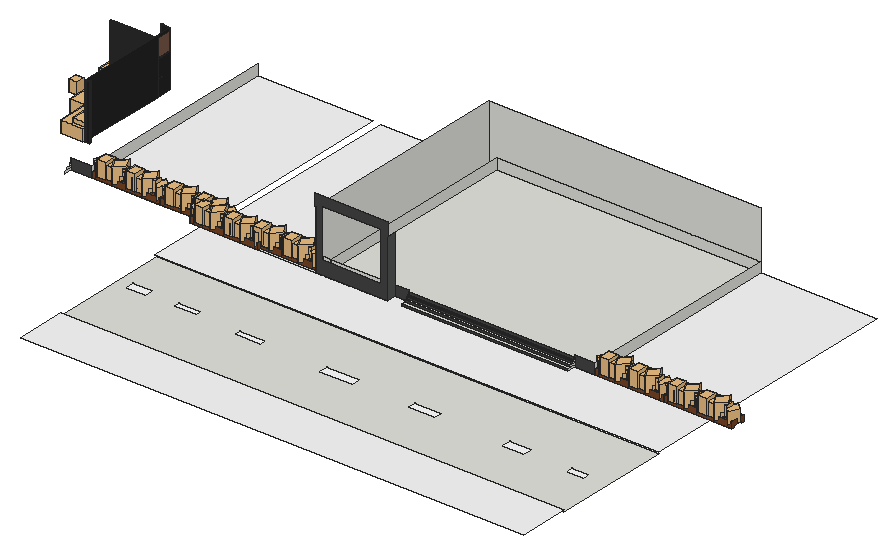
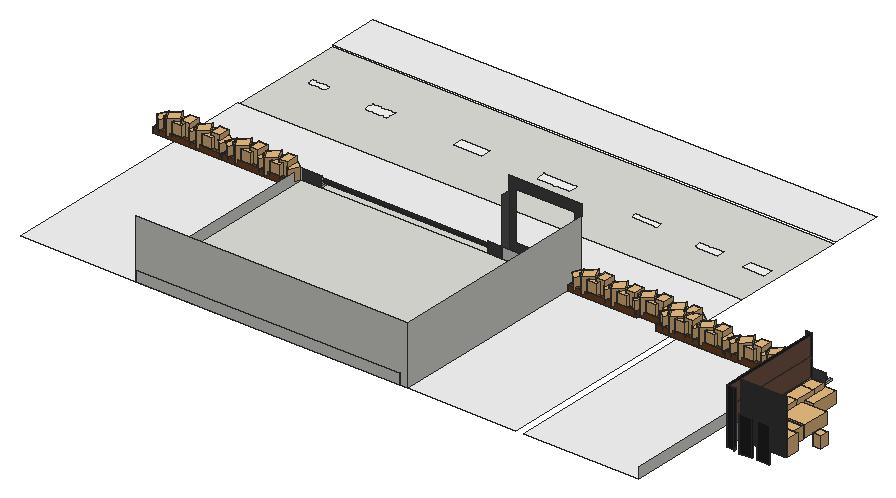
# SketchUp Ruby script. Lengths in inches.
U = 1.inch
M = Sketchup.active_model
def pt(a) = Geom::Point3d.new(a.map { |v| v * U })
def face(e, loops, mat)
  f = e.add_face(loops[0].map { |a| pt(a) })
  loops[1..].each { |l| e.add_face(l.map { |a| pt(a) }).erase! }
  f.material = f.back_material = mat if mat
  f
end
# faces: each face lists its corners as indices into pts; further lists are holes
def faces(e, pts, list, mat = nil) = list.each { |f| face(e, (f[0].is_a?(Array) ? f : [f]).map { |l| l.map { |i| pts[i] } }, mat) }
# xy, xz, yz: faces in a plane at the given z, y or x. An outline is a flat list of corners, or four numbers for a rectangle; further outlines are holes
def ring(l) = l.size == 4 ? [[l[0], l[1]], [l[2], l[1]], [l[2], l[3]], [l[0], l[3]]] : l.each_slice(2).to_a
def flat(e, list, mat, &to3) = list.each { |f| face(e, (f[0].is_a?(Array) ? f : [f]).map { |l| ring(l).map { |u, v| to3.(u, v) } }, mat) }
def xy(e, z, list, mat = nil) = flat(e, list, mat) { |x, y| [x, y, z] }
def xz(e, y, list, mat = nil) = flat(e, list, mat) { |x, z| [x, y, z] }
def yz(e, x, list, mat = nil) = flat(e, list, mat) { |y, z| [x, y, z] }
def lines(e, pts, list) = list.each { |a, b| e.add_line(pt(pts[a]), pt(pts[b])) }
# prism: a flat outline (further loops are holes) pulled along v
def prism(e, loops, v, mat = nil)
  f = face(e, loops, mat); d = Geom::Vector3d.new(v.map { |x| x * U })
  f.pushpull(f.normal.samedirection?(d) ? d.length : -d.length)
end
def box(e, o, s, mat = nil) = prism(e, [[o, [o[0] + s[0], o[1], o[2]], [o[0] + s[0], o[1] + s[1], o[2]], [o[0], o[1] + s[1], o[2]]]], [0, 0, s[2]], mat)
def at(x, y, z, deg = 0) = Geom::Transformation.translation(pt([x, y, z])) * Geom::Transformation.rotation(ORIGIN, Z_AXIS, deg.degrees)
def axes(o, x, y, z) = Geom::Transformation.new([*x, 0, *y, 0, *z, 0, *pt(o).to_a, 1])
def part(name) = M.definitions.add(name)
# library, detail: a bought-in or finely detailed component or shape, given as its bounding box
def library(name, o, s) = part(name).tap { |d| box(d.entities, o, s) }
def detail(e, o, s) = box(e.add_group.entities, o, s)
def put(e, d, t, mat = nil) = e.add_instance(d, t).tap { |i| i.material = mat if mat }
def group(e, t, mat = nil) = e.add_group.tap { |g| g.transformation = t; g.material = mat if mat }.entities
root = M.entities
M.materials.add("Aluminum_Polished").color = [83, 85, 85]
M.materials.add("Color_").color = [255, 255, 255]
M.materials.add("Floor board").color = [119, 86, 70]
M.materials.add("Floor board2").color = [119, 86, 70]
M.materials.add("Material__1").color = [95, 70, 46]
M.materials.add("Screen Shot 2014-10-30 at 12.13.07").color = [162, 155, 149]
M.materials.add("Sophie_Shoes2").color = [35, 35, 35]
M.materials.add("Untitsled-1").color = [96, 91, 93]
M.materials.add("Wood_Grain_Dark").color = [51, 47, 43]
M.materials.add("[Granite Dark Gray]").color = [69, 68, 68]
M.materials.add("[Metal_Corrogated_Shiny]2").color = [193, 193, 193]
M.materials.add("[Tile Grey]").color = [249, 249, 249]
M.materials.add("[Wood Veneer 01]").color = [120, 70, 37]
c1 = library("ch24 wishbone chair by Carl Hansen & Son",[0,0,0],[21.1,19.68,29.02])
c2 = part("Group\#72")
box(c2.entities,[0,-0.59,0],[31.5,1.77,87.4],"Sophie_Shoes2")
c3 = library("Armless sofa",[0,0,0],[31.59,51.18,39.76])
c4 = library("Sofa corner unit",[0,0,0],[31.57,31.52,39.76])
c5 = part("Group\#13")
box(c5.entities,[-0.79,0,0],[1.97,3.15,131.5],"Wood_Grain_Dark")
c6 = library("Group\#91",[-37.8,-0.03,0],[93.74,69.5,29.53])
c7 = library("Group\#68",[-37.8,-0.03,0],[93.74,69.5,29.53])
c8 = library("Group\#95",[0,-0.03,0],[55.94,69.5,29.53])
c9 = library("Areca palm plant",[0,0,0],[49.1,36.6,54.46])
c10 = library("Group\#440",[-84.69,-90.07,-0.36],[176.51,175.13,171.4])
c11 = library("Group\#441",[-7.34,-1.2,0],[38.67,35.81,49.04])
c12 = library("Group38\#2",[14.01,28.44,-23.43],[18.58,18.32,38.89])
c13 = library("Group20\#1",[-20.81,-17.08,3.79],[39.86,39.43,37.51])
c14 = part("Group\#443")
put(c14.entities,c9,axes([76.39,-6.2,6.08],[0.56191,0.45017,0],[-0.52986,0.66137,0],[0,0,0.72]))
put(c14.entities,c9,axes([178.2,-6.2,6.08],[0.56191,0.45017,0],[-0.52986,0.66137,0],[0,0,0.72]))
put(c14.entities,c10,axes([163.5,14.93,6.05],[0.08593,-0.04961,0],[0.04961,0.08593,0],[0,0,0.10522]))
put(c14.entities,c11,axes([144.89,24.9375,8],[-0.79,0,0],[0,-0.79,0],[0,0,0.79]))
put(c14.entities,c10,axes([113.57,17.19,6.07],[0.14087,-0.08133,0],[0.08133,0.14087,0],[0,0,0.1725]))
put(c14.entities,c12,axes([235.95,-4.1,28.17],[0,0.8848,0],[-0.94674,0,0],[0,0,0.85826]))
put(c14.entities,c10,axes([190.75,14.93,6.05],[0.08593,-0.04961,0],[0.04961,0.08593,0],[0,0,0.10522]))
put(c14.entities,c10,axes([61.68,14.93,6.05],[0.08593,-0.04961,0],[0.04961,0.08593,0],[0,0,0.10522]))
put(c14.entities,c10,axes([88.93,14.93,6.05],[0.08593,-0.04961,0],[0.04961,0.08593,0],[0,0,0.10522]))
put(c14.entities,c13,axes([154.82,18.97,4.77],[-0.85,0,0],[0,-0.85,0],[0,0,0.85]))
put(c14.entities,c10,axes([41.62,14.93,6.05],[0.08593,-0.04961,0],[0.04961,0.08593,0],[0,0,0.10522]))
put(c14.entities,c10,axes([143.43,14.93,6.05],[0.08593,-0.04961,0],[0.04961,0.08593,0],[0,0,0.10522]))
put(c14.entities,c12,axes([134.14,-4.1,28.17],[0,0.8848,0],[-0.94674,0,0],[0,0,0.85826]))
g1 = group(c14.entities,at(234.8,0,0,90),"[Wood Veneer 01]")
xy(g1,0,[[0,0,6,234.8],[30,0,36,234.8]])
xy(g1,3,[[6,0,30,234.8]])
xy(g1,7,[[6,5,30,229.8]],"Material__1")
xy(g1,15,[[[0,0,36,234.8],[6,5,30,229.8]]])
xz(g1,0,[[0,0,6,0,6,3,30,3,30,0,36,0,36,15,0,15]])
xz(g1,5,[[6,7,30,15]])
xz(g1,229.8,[[6,7,30,15]])
xz(g1,234.8,[[0,0,0,15,36,15,36,0,30,0,30,3,6,3,6,0]])
yz(g1,0,[[0,0,234.8,15]])
yz(g1,6,[[0,0,234.8,3],[5,7,229.8,15]])
yz(g1,30,[[0,0,234.8,3],[5,7,229.8,15]])
yz(g1,36,[[0,0,234.8,15]])
put(c14.entities,c11,axes([43.08,24.9375,8],[-0.79,0,0],[0,-0.79,0],[0,0,0.79]))
put(c14.entities,c10,axes([11.76,17.19,6.07],[0.14087,-0.08133,0],[0.08133,0.14087,0],[0,0,0.1725]))
put(c14.entities,c13,axes([53.01,18.97,4.77],[-0.85,0,0],[0,-0.85,0],[0,0,0.85]))
put(c14.entities,c10,axes([219.01,17.19,6.07],[0.14087,-0.08133,0],[0.08133,0.14087,0],[0,0,0.1725]))
c15 = part("Untitled (5)")
xy(c15.entities,0,[[[158.81,26.5625,306.06,993.3125],[226.57,518.17,239.57,583.92],[225.28,357.51,237.28,411.51],[222.61,182.28,236.36,226.53],[239.71,931.55,251.46,972.3],[233.64,703.93,242.14,755.18],[240.05,835.03,248.8,880.53],[222.04,66.5,231.29,100.5]]])
xy(c15.entities,0,[[222.04,66.5,231.29,100.5],[222.61,182.28,236.36,226.53],[225.28,357.51,237.28,411.51],[226.57,518.17,239.57,583.92],[233.64,703.93,242.14,755.18],
  [240.05,835.03,248.8,880.53],[239.71,931.55,251.46,972.3]],"Color_")
xy(root,-20.5,[[3778.5,559.875,4065.56,581.125],[4065.56,559.875,4244.09,581.125],[4279.08,559.875,4690.96,581.125],[4065.56,581.125,4085.31,1096.5],[4085.31,581.125,4742.06,1096.5]])
xy(root,-20.5,[[3778.5,419.4375,5029.12,419.4375,5029.12,581.125,4690.96,581.125,4690.96,559.875,4279.08,559.875,4279.08,581.125,4244.09,581.125,4244.09,559.875,3778.5,559.875],[3491.44,581.125,3778.5,1096.5],[3798.25,581.125,4065.56,1096.5],[4742.06,581.125,5029.12,1096.5]],"[Tile Grey]")
xy(root,-20.25,[[3778.5,0,5029.12,126.25]],"[Tile Grey]")
xy(root,-15.38,[[4279.08,559.875,4690.96,568.25]])
xy(root,-10.73,[[4279.08,568.25,4690.96,575.4375]])
xy(root,-6.62,[[4279.08,575.4375,4690.96,578]])
xy(root,-3.61,[[4279.08,578,4690.96,580.3125]])
xz(root,559.875,[[[4065.56,-20.5,4244.09,-20.5,4244.09,155.3125,4061.87,155.3125,4061.87,126,4065.56,126],[4079.48,11.5,4226.29,132]],[4279.08,-20.5,4690.96,-15.38]],"[Granite Dark Gray]")
xz(root,568.25,[[4279.08,-15.38,4690.96,-10.73]],"[Granite Dark Gray]")
xz(root,575.4375,[[4279.08,-10.73,4690.96,-6.62]],"[Granite Dark Gray]")
xz(root,578,[[4279.08,-6.62,4690.96,-3.61]],"[Granite Dark Gray]")
xz(root,580.3125,[[4279.08,-3.61,4690.96,1.19]],"[Granite Dark Gray]")
xz(root,581.125,[[4065.56,-20.5,4085.31,6],[4085.31,-20.5,4244.09,6]])
xz(root,581.125,[[3440.34,-20.5,3491.44,6],[4244.09,-20.5,4279.08,6],[4690.96,-20.5,4742.06,6]],"[Granite Dark Gray]")
xz(root,1096.5,[[4065.56,-20.5,4065.56,126,4742.06,126,4742.06,6,4085.31,6,4085.31,-20.5],[4085.31,-20.5,4742.06,6]])
yz(root,3440.34,[[559.875,-20.5,581.125,-15.38],[568.25,-15.38,581.125,-10.73],[575.4375,-10.73,581.125,-6.62],[578,-6.62,581.125,-3.61],[580.3125,-3.61,581.125,1.19]])
yz(root,3491.44,[[581.125,-20.5,1096.5,6]])
yz(root,4065.56,[[559.875,-20.5,581.125,6],[581.125,-20.5,581.125,6,559.875,6,559.875,126,1096.5,126,1096.5,-20.5]])
yz(root,4085.31,[[581.125,-20.5,1096.5,6]])
yz(root,4244.09,[[559.875,-20.5,581.125,120.25]],"Aluminum_Polished")
yz(root,4279.08,[[559.875,-20.5,581.125,-15.38],[568.25,-15.38,581.125,-10.73],[575.4375,-10.73,581.125,-6.62],[578,-6.62,581.125,-3.61],[580.3125,-3.61,581.125,1.19]])
yz(root,4690.96,[[559.875,-20.5,581.125,-15.38],[568.25,-15.38,581.125,-10.73],[575.4375,-10.73,581.125,-6.62],[578,-6.62,581.125,-3.61],[580.3125,-3.61,581.125,1.19]])
yz(root,4742.06,[[581.125,-20.5,1096.5,6]])
p = [[3345.91,994.6,0],[3345.91,994.79,0],[3427.37,658.2,0],[3427.4,658.2,0],[3414.37,657.34,0],[3414.37,657.34,86.61]]
lines(root,p,[[0,1],[2,3],[4,5]])
put(root,c1,axes([3266.16,790.81,0],[-0.00287,1,0],[1,0.00287,0],[0,0,1]))
put(root,c2,at(3304.21,923.74,0))
g2 = group(root,at(3325.58,648.625,-0.2))
put(g2,c3,at(86.72,196.88,0,-180))
put(g2,c3,at(86.72,145.7,0,-180))
put(g2,c3,at(4.02,228.45,0,-90))
put(g2,c4,at(55.2,228.45,0,-90))
put(g2,c4,at(86.72,43.34,0,-180))
put(g2,c4,at(-27.56,196.93,0))
put(g2,c3,at(86.72,94.52,0,-180))
g3 = group(root,at(3302.98,877.28,0))
put(g3,c5,at(100,0,0))
put(g3,c5,at(57.48,0,0))
put(g3,c5,at(92.91,0,0))
put(g3,c5,at(7.875,0,0))
put(g3,c5,at(107.09,0,0))
put(g3,c5,at(103.54,0,0))
put(g3,c5,at(61.02,0,0))
put(g3,c5,at(29.13,0,0))
put(g3,c5,at(68.11,0,0))
put(g3,c5,at(22.05,0,0))
put(g3,c5,at(78.74,0,0))
put(g3,c5,at(14.96,0,0))
put(g3,c5,at(82.28,0,0))
put(g3,c5,at(71.65,0,0))
put(g3,c5,at(75.2,0,0))
put(g3,c5,at(25.59,0,0))
put(g3,c5,at(18.5,0,0))
put(g3,c5,at(43.31,0,0))
put(g3,c5,at(64.57,0,0))
put(g3,c5,at(53.9375,0,0))
put(g3,c5,at(85.83,0,0))
put(g3,c5,at(89.37,0,0))
put(g3,c5,at(11.42,0,0))
put(g3,c5,at(0.79,0,0))
put(g3,c5,at(4.33,0,0))
put(g3,c5,at(36.22,0,0))
put(g3,c5,at(39.76,0,0))
put(g3,c5,at(32.68,0,0))
put(g3,c5,at(96.46,0,0))
put(g3,c5,at(46.85,0,0))
put(g3,c5,at(50.39,0,0))
put(g3,c5,at(-2.76,0,0))
put(root,c2,at(3348.06,923.74,0))
put(root,c6,at(3355.96,729.5,-0.2))
put(root,c7,at(3355.96,804.34,-0.2))
put(root,c8,at(3355.96,653.6,-0.2))
g4 = group(root,at(3397.45,657.41,0),"Sophie_Shoes2")
xy(g4,0,[[16.91,-1.18,16.91,-0.07,14.95,-0.07,14.95,222.49,16.91,222.49,16.91,261.27,-5.31,261.27,-5.31,266.33,-3.9375,266.33,-3.9375,262.65,17.7,262.65,17.7,223.02,18.5,223.02,18.5,0.79,29.91,0.79,29.95,0,29.95,-1.18]])
xy(g4,7.875,[[-5.31,261.27,-4.72,266.33],[-4.72,261.27,16.91,261.86]],"Untitsled-1")
xy(g4,36.61,[[15.34,0.32,16.91,222.1]])
xy(g4,39.37,[[14.95,-0.07,16.91,-0.07,16.91,0,17.7,0,17.7,261.86,16.91,261.86,16.91,0.32,15.34,0.32,15.34,222.1,16.91,222.1,16.91,222.49,14.95,222.49]])
xy(g4,40.55,[[16.91,0,17.7,223.02],[16.91,223.02,17.7,261.86]])
xy(g4,85.43,[[16.91,0,17.7,261.86]],"Floor board2")
xy(g4,86.61,[[16.91,0,17.7,261.86]])
xy(g4,131.5,[[16.91,-0.07,17.7,261.86]],"Floor board2")
xy(g4,137.8,[[17.7,-1.18,29.95,-1.18,29.95,0,29.91,0.79,18.5,0.79,18.5,223.02,17.7,223.02],[-4.72,261.86,17.7,261.86,17.7,262.65,-3.9375,262.65,-3.9375,266.33,-4.72,266.33]])
xy(g4,137.8,[[16.91,-1.18,17.7,-0.07]],"Sophie_Shoes2")
xz(g4,-1.18,[[16.91,0,29.95,137.8]],"Sophie_Shoes2")
xz(g4,-0.07,[[14.95,3.9375,16.91,39.37],[16.91,131.5,17.7,137.8]],"Sophie_Shoes2")
xz(g4,-0.07,[[14.95,0,16.91,3.9375]],"[Metal_Corrogated_Shiny]2")
xz(g4,0,[[16.91,39.37,17.7,40.55],[16.91,40.55,17.7,40.94],[16.91,85.43,17.7,86.61]])
xz(g4,0.32,[[15.34,36.61,16.52,39.37],[16.52,36.61,16.91,39.37]])
xz(g4,0.79,[[18.5,0,29.91,137.8]])
xz(g4,222.1,[[15.34,36.61,16.91,39.37]])
xz(g4,222.49,[[14.95,0,16.91,7.875],[14.95,7.875,16.91,39.37]],"Sophie_Shoes2")
xz(g4,261.27,[[-5.31,0,16.91,7.875]],"Untitsled-1")
xz(g4,261.86,[[16.91,39.37,17.7,39.76]])
xz(g4,261.86,[[-4.72,7.875,16.91,7.875,16.91,39.76,17.7,39.76,17.7,40.55,16.91,40.55,16.91,85.43,17.7,85.43,17.7,86.61,16.91,86.61,16.91,131.5,17.7,131.5,17.7,137.8,-4.72,137.8]],"Sophie_Shoes2")
xz(g4,262.65,[[-3.9375,0,17.7,137.8]])
xz(g4,266.33,[[-5.31,0,-5.31,7.875,-4.72,7.875,-4.72,137.8,-3.9375,137.8,-3.9375,0]])
yz(g4,-5.31,[[261.27,0,266.33,7.875]],"Untitsled-1")
yz(g4,-4.72,[[261.86,7.875,266.33,137.8]],"Sophie_Shoes2")
yz(g4,-3.9375,[[262.65,0,266.33,137.8]])
yz(g4,14.95,[[-0.07,3.9375,222.49,39.37]],"Sophie_Shoes2")
yz(g4,14.95,[[-0.07,0,222.49,3.9375]],"[Metal_Corrogated_Shiny]2")
yz(g4,15.34,[[0.32,36.61,222.1,39.37]])
yz(g4,16.91,[[0.32,36.61,222.1,39.37]])
yz(g4,16.91,[[0,40.55,0,40.94,-0.07,40.94,-0.07,86.61,0,86.61,0,85.43,261.86,85.43,261.86,40.55]],"Floor board")
yz(g4,16.91,[[-0.07,39.37,0,40.94],[-0.07,86.61,-0.07,131.5,261.86,131.5,261.86,87.4,232.86,87.4,232.86,86.61]],"Floor board2")
yz(g4,16.91,[[222.49,0,222.49,39.37,261.86,39.37,261.86,7.875,261.27,7.875,261.27,0]],"Screen Shot 2014-10-30 at 12.13.07")
yz(g4,16.91,[[-1.18,0,-0.07,40.94],[-1.18,40.94,-0.07,86.61],[-1.18,86.61,-0.07,137.8],[232.86,86.61,261.86,87.4]],"Sophie_Shoes2")
yz(g4,17.7,[[223.02,0,262.65,0,262.65,137.8,261.86,137.8,261.86,85.43,223.02,85.43,223.02,40.55,261.86,40.55,261.86,39.37,223.02,39.37],[0,39.37,261.86,40.55],[0,40.55,223.02,40.94],[0,85.43,261.86,86.61]])
yz(g4,17.7,[[-0.07,131.5,261.86,137.8]],"Sophie_Shoes2")
yz(g4,18.5,[[0.79,0,223.02,137.8]])
yz(g4,29.95,[[-1.18,0,0,137.8]])
p = [[29.95,0,0],[29.91,0.79,0],[29.91,0.79,137.8],[29.95,0,137.8],[16.91,261.86,105.12],[16.91,272.94,105.12],
  [16.91,49.92,72.44],[17.7,49.92,72.44],[16.91,0,72.44],[17.7,0,72.44],[17.7,0,105.12],[17.7,0.79,105.12],
  [16.91,49.92,105.12],[17.7,49.92,105.12],[16.91,0,105.12],[17.7,0.79,72.44],[16.52,0.32,39.37],[16.52,0.39,39.37],
  [17.31,0.39,39.37],[17.31,222.1,39.37],[17.31,261.47,39.37],[17.31,223.02,39.37],[16.91,222.1,39.37]]
faces(g4,p,[[0,1,2,3]])
lines(g4,p,[[4,5],[6,7],[8,9],[10,11],[12,13],[14,10],[15,7],[9,15],[16,17],[18,19],[20,21],[19,22],
  [21,19]])
put(root,c14,axes([3491.44,581.125,-20.5],[0.72468,0,0],[0,1,0],[0,0,1]))
put(root,c14,axes([3661.59,581.125,-20.5],[0.72468,0,0],[0,1,0],[0,0,1]))
put(root,c14,axes([3751.875,559.875,-20.5],[0.72468,0,0],[0,1,0],[0,0,1]))
put(root,c14,axes([3892.47,566.07,-20.5],[0.72468,0,0],[0,1,0],[0,0,1]))
put(root,c15,axes([5063.39,-189.95,-24.3125],[0,1.99109,0],[-1.29,0,0],[0,0,1.29]))
put(root,c14,axes([4742.06,581.125,-20.5],[0.72468,0,0],[0,1,0],[0,0,1]))
put(root,c14,axes([4912.21,581.125,-20.5],[0.72468,0,0],[0,1,0],[0,0,1]))
